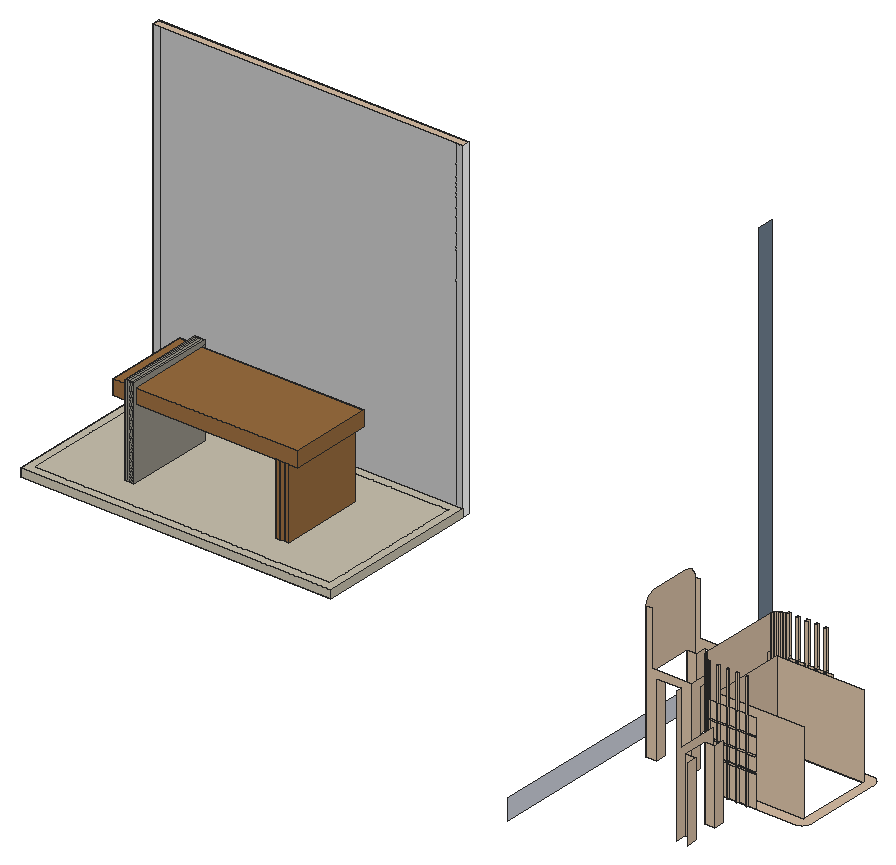
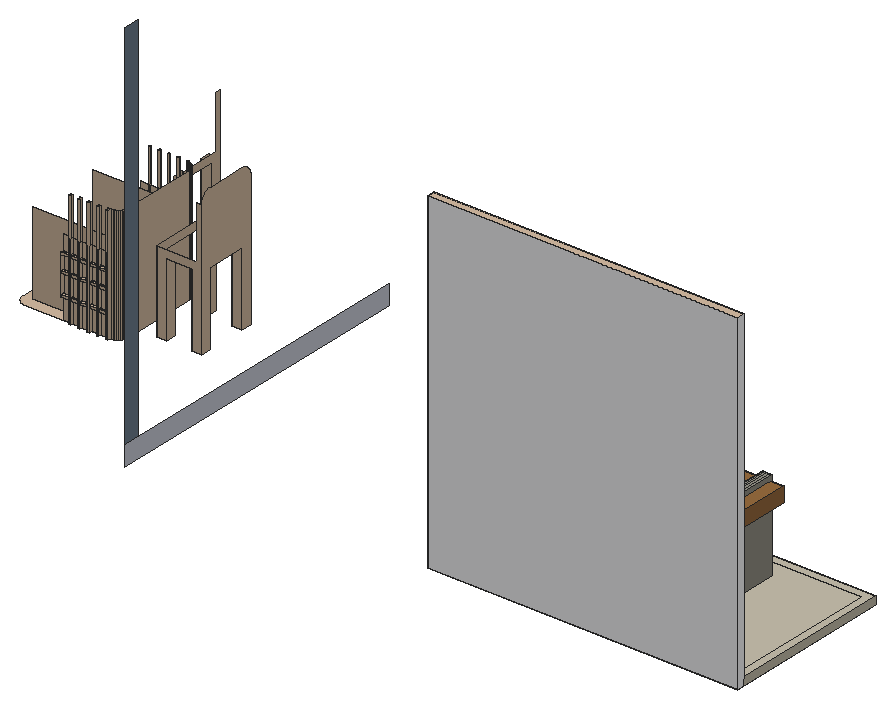
# SketchUp Ruby script. Lengths in inches.
U = 1.inch
M = Sketchup.active_model
def pt(a) = Geom::Point3d.new(a.map { |v| v * U })
def face(e, loops, mat)
  f = e.add_face(loops[0].map { |a| pt(a) })
  loops[1..].each { |l| e.add_face(l.map { |a| pt(a) }).erase! }
  f.material = f.back_material = mat if mat
  f
end
# faces: each face lists its corners as indices into pts; further lists are holes
def faces(e, pts, list, mat = nil) = list.each { |f| face(e, (f[0].is_a?(Array) ? f : [f]).map { |l| l.map { |i| pts[i] } }, mat) }
# xy, xz, yz: faces in a plane at the given z, y or x. An outline is a flat list of corners, or four numbers for a rectangle; further outlines are holes
def ring(l) = l.size == 4 ? [[l[0], l[1]], [l[2], l[1]], [l[2], l[3]], [l[0], l[3]]] : l.each_slice(2).to_a
def flat(e, list, mat, &to3) = list.each { |f| face(e, (f[0].is_a?(Array) ? f : [f]).map { |l| ring(l).map { |u, v| to3.(u, v) } }, mat) }
def xy(e, z, list, mat = nil) = flat(e, list, mat) { |x, y| [x, y, z] }
def xz(e, y, list, mat = nil) = flat(e, list, mat) { |x, z| [x, y, z] }
def yz(e, x, list, mat = nil) = flat(e, list, mat) { |y, z| [x, y, z] }
def lines(e, pts, list) = list.each { |a, b| e.add_line(pt(pts[a]), pt(pts[b])) }
# prism: a flat outline (further loops are holes) pulled along v
def prism(e, loops, v, mat = nil)
  f = face(e, loops, mat); d = Geom::Vector3d.new(v.map { |x| x * U })
  f.pushpull(f.normal.samedirection?(d) ? d.length : -d.length)
end
def box(e, o, s, mat = nil) = prism(e, [[o, [o[0] + s[0], o[1], o[2]], [o[0] + s[0], o[1] + s[1], o[2]], [o[0], o[1] + s[1], o[2]]]], [0, 0, s[2]], mat)
def at(x, y, z, deg = 0) = Geom::Transformation.translation(pt([x, y, z])) * Geom::Transformation.rotation(ORIGIN, Z_AXIS, deg.degrees)
def axes(o, x, y, z) = Geom::Transformation.new([*x, 0, *y, 0, *z, 0, *pt(o).to_a, 1])
def part(name) = M.definitions.add(name)
# library, detail: a bought-in or finely detailed component or shape, given as its bounding box
def library(name, o, s) = part(name).tap { |d| box(d.entities, o, s) }
def detail(e, o, s) = box(e.add_group.entities, o, s)
def put(e, d, t, mat = nil) = e.add_instance(d, t).tap { |i| i.material = mat if mat }
def group(e, t, mat = nil) = e.add_group.tap { |g| g.transformation = t; g.material = mat if mat }.entities
root = M.entities
M.materials.add("Cherry Matte 300cm").color = [152, 108, 63]
M.materials.add("Cherry Matte 300cm\#1").color = [152, 108, 63]
M.materials.add("[0111_SlateGray]").color = [112, 128, 144]
M.materials.add("[0131_Silver]").color = [192, 192, 192]
M.materials.add("[Formica Graystone]").color = [149, 146, 135]
M.materials.add("[Formica Laminate Light]").color = [213, 189, 164]
M.materials.add("[Marble Carrara Floor Tile]").color = [204, 208, 219]
M.materials.add("[Quartz Light Grey]").color = [251, 251, 252]
M.materials.add("[Tile Canvas]").color = [199, 192, 173]
xy(root,0,[[254.37,124.84,254.81,125.33],[257.68,124.84,258.11,125.33],[260.98,124.84,261.41,125.33],[264.28,124.84,264.71,125.33],[267.58,124.84,268.02,125.33],
  [[254.38,125.33,284.53,125.33,284.96,125.41,285.38,125.55,285.78,125.73,286.16,125.96,286.5,126.23,286.8125,126.55,287.08,126.89,287.31,127.27,287.49,127.67,287.62,128.09,287.69,128.53,287.72,128.96,287.72,155.08,287.7,155.54,287.62,155.99,287.49,156.43,287.32,156.86,287.1,157.26,286.83,157.63,286.53,157.98,286.1875,158.28,285.8125,158.55,285.41,158.77,284.99,158.95,284.55,159.08,254.38,159.08,253.88,159.05,253.4,158.94,252.93,158.76,252.49,158.52,252.09,158.22,251.74,157.87,251.45,157.47,251.21,157.03,251.04,156.5625,250.94,156.11,250.94,128.96,251.03,128.53,251.16,128.11,251.34,127.7,251.55,127.3125,251.81,126.95,252.09,126.61,252.42,126.3,252.77,126.03,253.14,125.79,253.54,125.6,253.95,125.44],[254.38,128.96,284.55,155.08]],[0,144.29,108,204.29],[241.57,147.05,245.21,150.5],[254.38,159.08,255.19,160.01],[257.64,159.08,258.46,160.01],
  [260.91,159.08,261.72,160.01],[264.17,159.08,264.98,160.01],[267.43,159.08,268.24,160.01]],"[Formica Laminate Light]")
xy(root,3.99,[[27.79,154.9,28.625,155.62],[28.625,154.9,29.46,155.62],[29.46,154.9,30.29,155.62],[30.29,154.9,31.125,155.62],[79.9,155.62,81.25,184.37],
  [81.25,155.62,82.71,184.37],[82.71,155.62,84.17,184.37],[27.79,184.37,28.625,185.45],[28.625,184.37,29.46,185.45],[29.46,184.37,30.29,185.45],
  [30.29,184.37,31.125,185.45]],"[Formica Laminate Light]")
xy(root,7.64,[[255.19,159.08,257.64,160.01],[258.46,159.08,260.91,160.01],[261.72,159.08,264.17,160.01],[264.98,159.08,267.43,160.01],[268.24,159.08,270.69,160.01]],"[Formica Laminate Light]")
xy(root,8.44,[[255.19,159.08,257.64,160.01],[258.46,159.08,260.91,160.01],[261.72,159.08,264.17,160.01],[268.24,159.08,270.69,160.01]],"[Formica Laminate Light]")
xy(root,8.46,[[264.98,159.08,267.43,160.01]],"[Formica Laminate Light]")
xy(root,11.02,[[254.81,124.84,257.68,125.33],[258.11,124.84,260.98,125.33],[261.41,124.84,264.28,125.33],[264.71,124.84,267.58,125.33],[268.02,124.84,270.89,125.33]],"[Formica Laminate Light]")
xy(root,11.55,[[254.81,124.84,257.68,125.33],[258.11,124.84,260.98,125.33],[261.41,124.84,264.28,125.33],[264.71,124.84,267.58,125.33],[268.02,124.84,270.89,125.33]],"[Formica Laminate Light]")
xy(root,15.1,[[255.19,159.08,257.64,160.01],[258.46,159.08,260.91,160.01],[261.72,159.08,264.17,160.01],[264.98,159.08,267.43,160.01],[268.24,159.08,270.69,160.01]],"[Formica Laminate Light]")
xy(root,15.9,[[255.19,159.08,257.64,160.01],[258.46,159.08,260.91,160.01],[268.24,159.08,270.69,160.01]],"[Formica Laminate Light]")
xy(root,15.91,[[261.72,159.08,264.17,160.01]],"[Formica Laminate Light]")
xy(root,15.92,[[264.98,159.08,267.43,160.01]],"[Formica Laminate Light]")
xy(root,16.52,[[254.81,124.84,257.68,125.33],[258.11,124.84,260.98,125.33],[261.41,124.84,264.28,125.33],[264.71,124.84,267.58,125.33],[268.02,124.84,270.89,125.33]],"[Formica Laminate Light]")
xy(root,20.88,[[255.19,159.08,257.64,160.01],[258.46,159.08,260.91,160.01],[261.72,159.08,264.17,160.01],[264.98,159.08,267.43,160.01],[268.24,159.08,270.69,160.01]],"[Formica Laminate Light]")
xy(root,21.68,[[255.19,159.08,257.64,160.01],[258.46,159.08,260.91,160.01],[261.72,159.08,264.17,160.01],[268.24,159.08,270.69,160.01]],"[Formica Laminate Light]")
xy(root,21.69,[[264.98,159.08,267.43,160.01]],"[Formica Laminate Light]")
xy(root,22.54,[[254.81,124.84,257.68,125.33],[258.11,124.84,260.98,125.33],[261.41,124.84,264.28,125.33],[264.71,124.84,267.58,125.33],[268.02,124.84,270.89,125.33]],"[Formica Laminate Light]")
xy(root,28.53,[[23.2,155.62,27.79,184.37]],"Cherry Matte 300cm")
xy(root,28.53,[[31.125,155.62,79.9,184.37],[84.17,155.62,87.4,184.37]],"Cherry Matte 300cm\#1")
xy(root,28.53,[[79.9,155.62,81.25,184.37]],"[Formica Laminate Light]")
xy(root,33.77,[[23.2,155.62,27.79,184.37],[31.125,155.62,87.4,184.37]],"Cherry Matte 300cm\#1")
xy(root,35.4,[[27.79,154.9,28.625,185.45],[28.625,154.9,29.46,185.45],[29.46,154.9,30.29,185.45],[30.29,154.9,31.125,185.45]],"[Formica Graystone]")
xy(root,115.75,[[0,201.68,108,204.29]],"[Formica Laminate Light]")
xz(root,101.59,[[265.27,0,268.91,25.5625]],"[Formica Laminate Light]")
xz(root,110.07,[[265.27,0,268.72,25.5625]],"[Formica Laminate Light]")
xz(root,124.84,[[254.37,0,254.81,40.33],[257.68,0,258.11,40.33],[260.98,0,261.41,40.33],[264.28,0,264.71,40.33],[267.58,0,268.02,40.33],
  [254.81,11.02,257.68,11.55],[258.11,11.02,260.98,11.55],[261.41,11.02,264.28,11.55],[264.71,11.02,267.58,11.55],[268.02,11.02,270.89,11.55],
  [254.81,16.52,257.68,17.06],[258.11,16.52,260.98,17.06],[261.41,16.52,264.28,17.06],[264.71,16.52,267.58,17.06],[268.02,16.52,270.89,17.06],
  [254.81,22.54,257.68,23.07],[258.11,22.54,260.98,23.07],[261.41,22.54,264.28,23.07],[264.71,22.54,267.58,23.07],[268.02,22.54,270.89,23.07]],"[Formica Laminate Light]")
xz(root,125.33,[[254.38,0,254.81,40.33],[254.81,0,257.68,11.02],[257.68,0,258.11,11.02],[258.11,0,260.98,11.02],[260.98,0,261.41,11.02],
  [261.41,0,264.28,11.02],[264.28,0,264.71,11.02],[264.71,0,267.58,11.02],[267.58,0,268.02,11.02],[268.02,0,270.89,11.02],
  [257.68,11.02,258.11,40.33],[260.98,11.02,261.41,40.33],[264.28,11.02,264.71,40.33],[267.58,11.02,268.02,40.33],[254.81,11.55,257.68,16.52],
  [258.11,11.55,260.98,16.52],[261.41,11.55,264.28,16.52],[264.71,11.55,267.58,16.52],[268.02,11.55,270.89,16.52],[254.81,16.52,257.68,22.54],
  [258.11,16.52,260.98,22.54],[261.41,16.52,264.28,22.54],[264.71,16.52,267.58,22.54],[268.02,16.52,270.89,22.54],[254.81,22.54,257.68,28.4],
  [258.11,22.54,260.98,28.4],[261.41,22.54,264.28,28.4],[264.71,22.54,267.58,28.4],[268.02,22.54,270.89,28.4]],"[Formica Laminate Light]")
xz(root,128.96,[[254.38,0,284.55,28.69]],"[Formica Laminate Light]")
xz(root,129.3,[[229.44,0,233.08,0,233.08,25.5625,241.57,25.5625,241.57,0,245.21,0,245.21,28.25,231.32,28.25,231.32,46.86,229.44,46.86]],"[Formica Laminate Light]")
xz(root,132.94,[[229.44,0,233.08,25.5625],[241.57,0,245.21,25.5625]],"[Formica Laminate Light]")
xz(root,146.86,[[229.44,0,233.08,25.5625]],"[Formica Laminate Light]")
xz(root,147.05,[[241.57,0,245.21,25.5625]],"[Formica Laminate Light]")
xz(root,150.5,[[229.44,0,229.44,46.75,231.32,46.75,231.32,28.25,245.21,28.25,245.21,0,241.57,0,241.57,25.5625,233.08,25.5625,233.08,0]],"[Formica Laminate Light]")
xz(root,154.9,[[27.79,3.99,28.625,35.4],[28.625,3.99,29.46,35.4],[29.46,3.99,30.29,35.4],[30.29,3.99,31.125,35.4]],"[Formica Graystone]")
xz(root,155.08,[[254.38,0,284.55,28.69]],"[Formica Laminate Light]")
xz(root,155.62,[[79.9,3.99,81.25,28.53],[81.25,3.99,82.71,28.53],[82.71,3.99,84.17,28.53],[23.2,28.53,27.79,33.77],[31.125,28.53,87.4,33.77]],"Cherry Matte 300cm\#1")
xz(root,159.08,[[254.38,0,255.19,40.33],[255.19,0,257.64,7.64],[257.64,0,258.46,40.33],[258.46,0,260.91,7.64],[260.91,0,261.72,40.33],
  [261.72,0,264.17,7.64],[264.17,0,264.98,40.33],[264.98,0,267.43,7.64],[267.43,0,268.24,40.33],[268.24,0,270.69,7.64],
  [255.19,8.44,257.64,15.1],[258.46,8.44,260.91,15.1],[261.72,8.44,264.17,15.1],[268.24,8.44,270.69,15.1],[264.98,8.46,267.43,15.1],
  [255.19,15.1,257.64,15.9],[258.46,15.1,260.91,15.9],[261.72,15.1,264.17,15.91],[264.98,15.1,267.43,15.92],[268.24,15.1,270.69,15.9],
  [255.19,15.9,257.64,20.88],[258.46,15.9,260.91,20.88],[268.24,15.9,270.69,20.88],[261.72,15.91,264.17,20.88],[264.98,15.92,267.43,20.88],
  [255.19,20.88,257.64,21.68],[258.46,20.88,260.91,21.68],[261.72,20.88,264.17,21.68],[264.98,20.88,267.43,21.69],[268.24,20.88,270.69,21.68],
  [255.19,21.68,257.64,26.83],[258.46,21.68,260.91,26.83],[261.72,21.68,264.17,26.83],[268.24,21.68,270.69,26.83],[264.98,21.69,267.43,26.83]],"[Formica Laminate Light]")
xz(root,160.01,[[254.38,0,255.19,40.33],[257.64,0,258.46,40.33],[260.91,0,261.72,40.33],[264.17,0,264.98,40.33],[267.43,0,268.24,40.33],
  [255.19,7.64,257.64,8.44],[258.46,7.64,260.91,8.44],[261.72,7.64,264.17,8.44],[264.98,7.64,267.43,8.46],[268.24,7.64,270.69,8.44],
  [255.19,15.1,257.64,15.9],[258.46,15.1,260.91,15.9],[261.72,15.1,264.17,15.91],[264.98,15.1,267.43,15.92],[268.24,15.1,270.69,15.9],
  [255.19,20.88,257.64,21.68],[258.46,20.88,260.91,21.68],[261.72,20.88,264.17,21.68],[264.98,20.88,267.43,21.69],[268.24,20.88,270.69,21.68]],"[Formica Laminate Light]")
xz(root,184.37,[[23.2,28.53,27.79,33.77],[31.125,28.53,87.4,33.77]],"Cherry Matte 300cm\#1")
xz(root,184.37,[[79.9,3.99,81.25,28.53],[81.25,3.99,82.71,28.53],[82.71,3.99,84.17,28.53]],"[Formica Laminate Light]")
xz(root,185.45,[[27.79,3.99,28.625,35.4],[28.625,3.99,29.46,35.4],[29.46,3.99,30.29,35.4],[30.29,3.99,31.125,35.4]],"[Formica Graystone]")
xz(root,201.68,[[0,2.75,2.61,115.75]],"[0131_Silver]")
yz(root,23.2,[[155.62,28.53,184.37,33.77]],"Cherry Matte 300cm\#1")
yz(root,27.79,[[[154.9,3.99,185.45,35.4],[155.62,28.53,184.37,33.77]]],"[Formica Graystone]")
yz(root,31.125,[[154.9,3.99,185.45,3.99,185.45,28.53,155.62,28.53,155.62,33.77,185.45,33.77,185.45,35.4,154.9,35.4],[184.37,28.53,185.45,33.77]],"[Formica Graystone]")
yz(root,79.9,[[155.62,3.99,184.37,28.53]],"Cherry Matte 300cm\#1")
yz(root,81.25,[[155.62,3.99,184.37,28.53]],"[Formica Laminate Light]")
yz(root,82.71,[[155.62,3.99,184.37,28.53]],"[Formica Laminate Light]")
yz(root,84.17,[[155.62,3.99,184.37,28.53]],"Cherry Matte 300cm\#1")
yz(root,87.4,[[155.62,28.53,184.37,33.77]],"Cherry Matte 300cm\#1")
yz(root,214.53,[[197,0,202.625,129.75]],"[0111_SlateGray]")
yz(root,214.53,[[88,-6.9375,202.625,0]],"[Marble Carrara Floor Tile]")
yz(root,229.44,[[129.3,0,129.3,46.86,129.36,47.34,129.48,47.8,129.65,48.25,129.89,48.67,130.17,49.05,130.5,49.4,130.87,49.71,131.27,49.97,131.7,50.17,132.16,50.32,132.63,50.41,133.11,50.4375,146.82,50.4375,147.3,50.41,147.77,50.3125,148.23,50.16,148.66,49.94,149.06,49.68,149.42,49.36,149.74,48.99,150.01,48.59,150.22,48.16,150.38,47.7,150.47,47.23,150.5,46.75,150.5,0,146.86,0,146.86,25.5625,132.94,25.5625,132.94,0]],"[Formica Laminate Light]")
yz(root,233.08,[[129.3,0,132.94,25.5625],[146.86,0,150.5,25.5625]],"[Formica Laminate Light]")
yz(root,241.57,[[129.3,0,132.94,25.5625],[147.05,0,150.5,25.5625]],"[Formica Laminate Light]")
yz(root,245.21,[[129.3,0,132.94,0,132.94,25.5625,147.05,25.5625,147.05,0,150.5,0,150.5,28.25,129.3,28.25]],"[Formica Laminate Light]")
yz(root,250.94,[[128.96,0,155.08,0,155.08,28.69,156.11,28.69,156.11,40.33,128.96,40.33],[155.08,0,156.11,28.69]],"[Formica Laminate Light]")
yz(root,254.37,[[124.84,0,125.33,40.33]],"[Formica Laminate Light]")
yz(root,254.38,[[128.96,0,155.08,28.69],[159.08,0,160.01,40.33]],"[Formica Laminate Light]")
yz(root,254.81,[[124.84,0,125.33,11.02],[124.84,11.02,125.33,11.55],[124.84,11.55,125.33,16.52],[124.84,16.52,125.33,22.54],[124.84,22.54,125.33,28.4]],"[Formica Laminate Light]")
yz(root,255.19,[[159.08,0,160.01,7.64],[159.08,7.64,160.01,8.44],[159.08,8.44,160.01,15.1],[159.08,15.1,160.01,15.9],[159.08,15.9,160.01,20.88],
  [159.08,20.88,160.01,21.68],[159.08,21.68,160.01,26.83]],"[Formica Laminate Light]")
yz(root,257.64,[[159.08,0,160.01,7.64],[159.08,7.64,160.01,8.44],[159.08,8.44,160.01,15.1],[159.08,15.1,160.01,15.9],[159.08,15.9,160.01,20.88],
  [159.08,20.88,160.01,21.68],[159.08,21.68,160.01,26.83]],"[Formica Laminate Light]")
yz(root,257.68,[[124.84,0,125.33,11.02],[124.84,11.02,125.33,11.55],[124.84,11.55,125.33,16.52],[124.84,16.52,125.33,22.54],[124.84,22.54,125.33,28.4]],"[Formica Laminate Light]")
yz(root,258.11,[[124.84,0,125.33,11.02],[124.84,11.02,125.33,11.55],[124.84,11.55,125.33,16.52],[124.84,16.52,125.33,22.54],[124.84,22.54,125.33,28.4]],"[Formica Laminate Light]")
yz(root,258.46,[[159.08,0,160.01,7.64],[159.08,7.64,160.01,8.44],[159.08,8.44,160.01,15.1],[159.08,15.1,160.01,15.9],[159.08,15.9,160.01,20.88],
  [159.08,20.88,160.01,21.68],[159.08,21.68,160.01,26.83]],"[Formica Laminate Light]")
yz(root,260.91,[[159.08,0,160.01,7.64],[159.08,7.64,160.01,8.44],[159.08,8.44,160.01,15.1],[159.08,15.1,160.01,15.9],[159.08,15.9,160.01,20.88],
  [159.08,20.88,160.01,21.68],[159.08,21.68,160.01,26.83]],"[Formica Laminate Light]")
yz(root,260.98,[[124.84,0,125.33,11.02],[124.84,11.02,125.33,11.55],[124.84,11.55,125.33,16.52],[124.84,16.52,125.33,22.54],[124.84,22.54,125.33,28.4]],"[Formica Laminate Light]")
yz(root,261.41,[[124.84,0,125.33,11.02],[124.84,11.02,125.33,11.55],[124.84,11.55,125.33,16.52],[124.84,16.52,125.33,22.54],[124.84,22.54,125.33,28.4]],"[Formica Laminate Light]")
yz(root,261.72,[[159.08,0,160.01,7.64],[159.08,7.64,160.01,8.44],[159.08,8.44,160.01,15.1],[159.08,15.1,160.01,15.91],[159.08,15.91,160.01,20.88],
  [159.08,20.88,160.01,21.68],[159.08,21.68,160.01,26.83]],"[Formica Laminate Light]")
yz(root,264.17,[[159.08,0,160.01,7.64],[159.08,7.64,160.01,8.44],[159.08,8.44,160.01,15.1],[159.08,15.1,160.01,15.91],[159.08,15.91,160.01,20.88],
  [159.08,20.88,160.01,21.68],[159.08,21.68,160.01,26.83]],"[Formica Laminate Light]")
yz(root,264.28,[[124.84,0,125.33,11.02],[124.84,11.02,125.33,11.55],[124.84,11.55,125.33,16.52],[124.84,16.52,125.33,22.54],[124.84,22.54,125.33,28.4]],"[Formica Laminate Light]")
yz(root,264.71,[[124.84,0,125.33,11.02],[124.84,11.02,125.33,11.55],[124.84,11.55,125.33,16.52],[124.84,16.52,125.33,22.54],[124.84,22.54,125.33,28.4]],"[Formica Laminate Light]")
yz(root,264.98,[[159.08,0,160.01,7.64],[159.08,7.64,160.01,8.46],[159.08,8.46,160.01,15.1],[159.08,15.1,160.01,15.92],[159.08,15.92,160.01,20.88],
  [159.08,20.88,160.01,21.69],[159.08,21.69,160.01,26.83]],"[Formica Laminate Light]")
yz(root,265.27,[[97.95,0,97.95,46.75,99.82,46.75,99.82,28.25,113.72,28.25,113.72,0,110.07,0,110.07,25.5625,101.59,25.5625,101.59,0]],"[Formica Laminate Light]")
yz(root,267.43,[[159.08,0,160.01,7.64],[159.08,7.64,160.01,8.46],[159.08,8.46,160.01,15.1],[159.08,15.1,160.01,15.92],[159.08,15.92,160.01,20.88],
  [159.08,20.88,160.01,21.69],[159.08,21.69,160.01,26.83]],"[Formica Laminate Light]")
yz(root,267.58,[[124.84,0,125.33,11.02],[124.84,11.02,125.33,11.55],[124.84,11.55,125.33,16.52],[124.84,16.52,125.33,22.54],[124.84,22.54,125.33,28.4]],"[Formica Laminate Light]")
yz(root,268.02,[[124.84,0,125.33,11.02],[124.84,11.02,125.33,11.55],[124.84,11.55,125.33,16.52],[124.84,16.52,125.33,22.54],[124.84,22.54,125.33,28.4]],"[Formica Laminate Light]")
yz(root,268.24,[[159.08,0,160.01,7.64],[159.08,7.64,160.01,8.44],[159.08,8.44,160.01,15.1],[159.08,15.1,160.01,15.9],[159.08,15.9,160.01,20.88],
  [159.08,20.88,160.01,21.68],[159.08,21.68,160.01,26.83]],"[Formica Laminate Light]")
yz(root,268.72,[[110.07,0,113.72,25.5625]],"[Formica Laminate Light]")
yz(root,268.91,[[97.95,0,101.59,25.5625]],"[Formica Laminate Light]")
yz(root,270.69,[[159.08,7.64,160.01,8.44],[159.08,8.44,160.01,15.1],[159.08,15.1,160.01,15.9],[159.08,15.9,160.01,20.88]],"[Formica Laminate Light]")
p = [[253.95,125.44,40.33],[253.95,125.44,0],[254.38,125.33,0],[254.38,125.33,40.33],[253.54,125.6,40.33],[253.54,125.6,0],
  [253.14,125.79,40.33],[253.14,125.79,0],[252.77,126.03,40.33],[252.77,126.03,0],[252.42,126.3,40.33],[252.42,126.3,0],
  [252.09,126.61,40.33],[252.09,126.61,0],[251.81,126.95,40.33],[251.81,126.95,0],[251.55,127.3125,40.33],[251.55,127.3125,0],
  [251.34,127.7,40.33],[251.34,127.7,0],[251.16,128.11,40.33],[251.16,128.11,0],[251.03,128.53,40.33],[251.03,128.53,0],
  [250.94,128.96,40.33],[250.94,128.96,0],[251.04,156.5625,40.33],[251.04,156.5625,0],[250.94,156.11,0],[250.94,156.11,28.69],
  [250.94,156.11,40.33],[251.21,157.03,40.33],[251.21,157.03,0],[251.45,157.47,40.33],[251.45,157.47,0],[251.74,157.87,40.33],
  [251.74,157.87,0],[252.09,158.22,40.33],[252.09,158.22,0],[252.49,158.52,40.33],[252.49,158.52,0],[252.93,158.76,40.33],
  [252.93,158.76,0],[253.4,158.94,40.33],[253.4,158.94,0],[253.88,159.05,40.33],[253.88,159.05,0],[254.38,159.08,40.33],
  [254.38,159.08,0]]
faces(root,p,[[0,1,2,3],[4,5,1,0],[6,7,5,4],[8,9,7,6],[10,11,9,8],[12,13,11,10],[14,15,13,12],[16,17,15,14],
  [18,19,17,16],[20,21,19,18],[22,23,21,20],[24,25,23,22],[26,27,28,29,30],[31,32,27,26],[33,34,32,31],[35,36,34,33],
  [37,38,36,35],[39,40,38,37],[41,42,40,39],[43,44,42,41],[45,46,44,43],[47,48,46,45]],"[Formica Laminate Light]")
g1 = group(root,at(0,144.29,0),"[Formica Laminate Light]")
xy(g1,2.75,[[[0,0,108,57.39],[2.61,2.61,105.39,54.58]],[2.61,2.61,105.39,54.58]],"[Tile Canvas]")
xz(g1,0,[[0,0,108,2.75]],"[Tile Canvas]")
yz(g1,0,[[0,0,57.39,2.75]],"[Tile Canvas]")
yz(g1,108,[[0,0,57.39,2.75]],"[Tile Canvas]")
g2 = group(root,at(0,201.68,0),"[Formica Laminate Light]")
xz(g2,0,[[2.61,2.75,105.39,115.75],[105.39,2.75,108,115.75]],"[0131_Silver]")
xz(g2,2.61,[[0,0,108,115.75]],"[Quartz Light Grey]")
yz(g2,0,[[0,0,2.61,115.75]],"[Quartz Light Grey]")
yz(g2,108,[[0,0,2.61,115.75]],"[Quartz Light Grey]")
